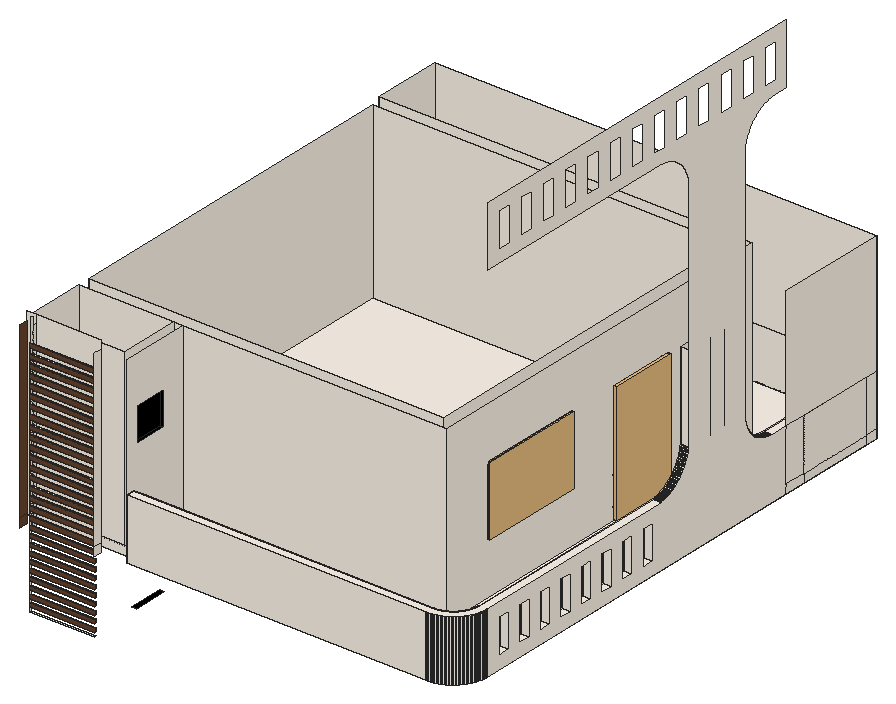
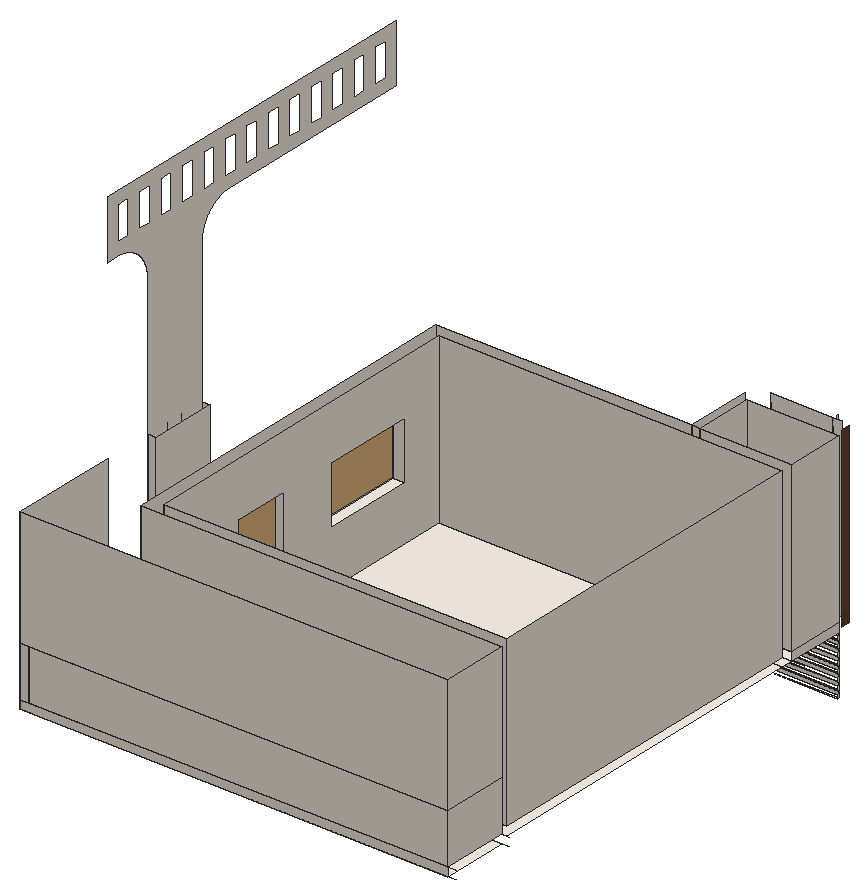
# SketchUp Ruby script. Lengths in inches.
U = 1.inch
M = Sketchup.active_model
def pt(a) = Geom::Point3d.new(a.map { |v| v * U })
def face(e, loops, mat)
  f = e.add_face(loops[0].map { |a| pt(a) })
  loops[1..].each { |l| e.add_face(l.map { |a| pt(a) }).erase! }
  f.material = f.back_material = mat if mat
  f
end
# faces: each face lists its corners as indices into pts; further lists are holes
def faces(e, pts, list, mat = nil) = list.each { |f| face(e, (f[0].is_a?(Array) ? f : [f]).map { |l| l.map { |i| pts[i] } }, mat) }
# xy, xz, yz: faces in a plane at the given z, y or x. An outline is a flat list of corners, or four numbers for a rectangle; further outlines are holes
def ring(l) = l.size == 4 ? [[l[0], l[1]], [l[2], l[1]], [l[2], l[3]], [l[0], l[3]]] : l.each_slice(2).to_a
def flat(e, list, mat, &to3) = list.each { |f| face(e, (f[0].is_a?(Array) ? f : [f]).map { |l| ring(l).map { |u, v| to3.(u, v) } }, mat) }
def xy(e, z, list, mat = nil) = flat(e, list, mat) { |x, y| [x, y, z] }
def xz(e, y, list, mat = nil) = flat(e, list, mat) { |x, z| [x, y, z] }
def yz(e, x, list, mat = nil) = flat(e, list, mat) { |y, z| [x, y, z] }
def lines(e, pts, list) = list.each { |a, b| e.add_line(pt(pts[a]), pt(pts[b])) }
# prism: a flat outline (further loops are holes) pulled along v
def prism(e, loops, v, mat = nil)
  f = face(e, loops, mat); d = Geom::Vector3d.new(v.map { |x| x * U })
  f.pushpull(f.normal.samedirection?(d) ? d.length : -d.length)
end
def box(e, o, s, mat = nil) = prism(e, [[o, [o[0] + s[0], o[1], o[2]], [o[0] + s[0], o[1] + s[1], o[2]], [o[0], o[1] + s[1], o[2]]]], [0, 0, s[2]], mat)
def at(x, y, z, deg = 0) = Geom::Transformation.translation(pt([x, y, z])) * Geom::Transformation.rotation(ORIGIN, Z_AXIS, deg.degrees)
def axes(o, x, y, z) = Geom::Transformation.new([*x, 0, *y, 0, *z, 0, *pt(o).to_a, 1])
def part(name) = M.definitions.add(name)
# library, detail: a bought-in or finely detailed component or shape, given as its bounding box
def library(name, o, s) = part(name).tap { |d| box(d.entities, o, s) }
def detail(e, o, s) = box(e.add_group.entities, o, s)
def put(e, d, t, mat = nil) = e.add_instance(d, t).tap { |i| i.material = mat if mat }
def group(e, t, mat = nil) = e.add_group.tap { |g| g.transformation = t; g.material = mat if mat }.entities
root = M.entities
M.materials.add("C01_Vanilla_Cream").color = [255, 246, 235]
M.materials.add("Wood_Veneer_15_1K").color = [103, 69, 45]
M.materials.add("[Color_009]1").color = [0, 0, 0]
c1 = library("porta+4",[0.2,-5.42,1.33],[46.55,4.72,83.21])
c2 = library("mesh-164",[-1582.71,-3144.16,-23.22],[2366.42,2227.34,65.81])
c3 = part("Group13")
put(c3.entities,c2,at(294.66,859.51,3.5))
xy(root,219.82,[[66,1,111,2]],"C01_Vanilla_Cream")
xy(root,222.5,[[66,1,111,2]],"C01_Vanilla_Cream")
xy(root,227.85,[[66,1,111,2]],"C01_Vanilla_Cream")
xy(root,230.52,[[66,1,111,2]],"C01_Vanilla_Cream")
xy(root,231,[[303,93,312,159],[303,201,312,243]],"C01_Vanilla_Cream")
xy(root,233.2,[[66,1,111,2]],"C01_Vanilla_Cream")
xy(root,235.875,[[66,1,111,2]],"C01_Vanilla_Cream")
xy(root,237.8,[[126,14.34,129,38.34]],"[Color_009]1")
xy(root,238.55,[[66,1,111,2]],"C01_Vanilla_Cream")
xy(root,241.22,[[66,1,111,2]],"C01_Vanilla_Cream")
xy(root,243.9,[[66,1,111,2]],"C01_Vanilla_Cream")
xy(root,246.58,[[66,1,111,2]],"C01_Vanilla_Cream")
xy(root,249.25,[[66,1,111,2]],"C01_Vanilla_Cream")
xy(root,251.92,[[66,1,111,2]],"C01_Vanilla_Cream")
xy(root,254.6,[[66,1,111,2]],"C01_Vanilla_Cream")
xy(root,257.27,[[66,1,111,2]],"C01_Vanilla_Cream")
xy(root,259.95,[[66,1,111,2]],"C01_Vanilla_Cream")
xy(root,262.625,[[66,1,111,2]],"C01_Vanilla_Cream")
xy(root,265.3,[[66,1,111,2]],"C01_Vanilla_Cream")
xy(root,267.98,[[66,1,111,2]],"C01_Vanilla_Cream")
xy(root,270,[[57,12,123,54],[123,12,129,54],[57,54,303,63],[303,54,312,318],[57,63,303,309],
  [54,318,303,366],[303,318,312,366]],"C01_Vanilla_Cream")
xy(root,270,[[129,6,129,54,312,54,312,366,360,366,360,30,359.99,29.25,359.95,28.49,359.89,27.74,359.8125,26.99,359.7,26.25,359.57,25.5,359.42,24.76,359.25,24.03,359.05,23.3,358.83,22.58,358.58,21.87,358.31,21.17,358.03,20.47,357.72,19.78,357.38,19.1,357.03,18.4375,356.66,17.78,356.26,17.14,355.85,16.51,355.42,15.89,354.96,15.29,354.49,14.7,354,14.13,353.5,13.57,352.97,13.03,352.43,12.5,351.87,12,351.3,11.51,350.71,11.04,350.11,10.58,349.49,10.15,348.86,9.74,348.22,9.34,347.5625,8.97,346.9,8.62,346.22,8.28,345.53,7.97,344.83,7.69,344.13,7.42,343.42,7.17,342.7,6.95,341.97,6.75,341.24,6.58,340.5,6.43,339.75,6.3,339.01,6.1875,338.26,6.11,337.51,6.05,336.75,6.01,336,6]],"Wood_Veneer_15_1K")
xy(root,270.65,[[66,1,111,2]],"C01_Vanilla_Cream")
xy(root,273.32,[[66,1,111,2]],"C01_Vanilla_Cream")
xy(root,276,[[66,1,111,2],[129,12,336,12,336.57,12.01,337.13,12.04,337.69,12.08,338.26,12.14,338.82,12.22,339.37,12.32,339.93,12.43,340.48,12.57,341.02,12.71,341.5625,12.88,342.1,13.0625,342.625,13.26,343.15,13.48,343.66,13.71,344.17,13.96,344.67,14.23,345.16,14.51,345.64,14.8,346.12,15.11,346.58,15.4375,347.03,15.78,347.47,16.13,347.9,16.5,348.32,16.88,348.73,17.27,349.12,17.68,349.5,18.1,349.87,18.53,350.22,18.97,350.5625,19.42,350.89,19.88,351.2,20.36,351.49,20.84,351.77,21.33,352.04,21.83,352.29,22.34,352.52,22.85,352.74,23.375,352.9375,23.9,353.12,24.4375,353.29,24.98,353.43,25.52,353.57,26.07,353.68,26.63,353.78,27.18,353.86,27.74,353.92,28.31,353.96,28.87,353.99,29.43,354,30,354,366,54,366,54,318,312,318,312,54,129,54],[57,12,123,54],[123,12,129,54],[57,63,303,309]],"C01_Vanilla_Cream")
xy(root,279,[[354,39,360,47.89],[354,56.78,360,65.67],[354,74.56,360,83.44],[354,92.33,360,101.22],[354,110.11,360,119],
  [354,127.89,360,136.78],[354,145.67,360,154.56],[354,163.44,360,172.33],[303,201,312,243]],"C01_Vanilla_Cream")
xy(root,279.15,[[66,1,111,2]],"C01_Vanilla_Cream")
xy(root,282.3,[[66,1,111,2]],"C01_Vanilla_Cream")
xy(root,285.45,[[66,1,111,2]],"C01_Vanilla_Cream")
xy(root,288.6,[[66,1,111,2]],"C01_Vanilla_Cream")
xy(root,291.75,[[66,1,111,2]],"C01_Vanilla_Cream")
xy(root,294.9,[[66,1,111,2]],"C01_Vanilla_Cream")
xy(root,298.05,[[66,1,111,2]],"C01_Vanilla_Cream")
xy(root,301.2,[[66,1,111,2]],"C01_Vanilla_Cream")
xy(root,303,[[354,39,360,47.89],[354,56.78,360,65.67],[354,74.56,360,83.44],[354,92.33,360,101.22],[354,110.11,360,119],
  [354,127.89,360,136.78],[354,145.67,360,154.56],[354,163.44,360,172.33]],"C01_Vanilla_Cream")
xy(root,304.35,[[66,1,111,2]],"C01_Vanilla_Cream")
xy(root,307.5,[[66,1,111,2]],"C01_Vanilla_Cream")
xy(root,310.65,[[66,1,111,2]],"C01_Vanilla_Cream")
xy(root,312,[[129,6,336,6,336.75,6.01,337.51,6.05,338.26,6.11,339.01,6.1875,339.75,6.3,340.5,6.43,341.24,6.58,341.97,6.75,342.7,6.95,343.42,7.17,344.13,7.42,344.83,7.69,345.53,7.97,346.22,8.28,346.9,8.62,347.5625,8.97,348.22,9.34,348.86,9.74,349.49,10.15,350.11,10.58,350.71,11.04,351.3,11.51,351.87,12,352.43,12.5,352.97,13.03,353.5,13.57,354,14.13,354.49,14.7,354.96,15.29,355.42,15.89,355.85,16.51,356.26,17.14,356.66,17.78,357.03,18.4375,357.38,19.1,357.72,19.78,358.03,20.47,358.31,21.17,358.58,21.87,358.83,22.58,359.05,23.3,359.25,24.03,359.42,24.76,359.57,25.5,359.7,26.25,359.8125,26.99,359.89,27.74,359.95,28.49,359.99,29.25,360,30,360,180,354,180,354,30,353.99,29.43,353.96,28.87,353.92,28.31,353.86,27.74,353.78,27.18,353.68,26.63,353.57,26.07,353.43,25.52,353.29,24.98,353.12,24.4375,352.9375,23.9,352.74,23.375,352.52,22.85,352.29,22.34,352.04,21.83,351.77,21.33,351.49,20.84,351.2,20.36,350.89,19.88,350.5625,19.42,350.22,18.97,349.87,18.53,349.5,18.1,349.12,17.68,348.73,17.27,348.32,16.88,347.9,16.5,347.47,16.13,347.03,15.78,346.58,15.4375,346.12,15.11,345.64,14.8,345.16,14.51,344.67,14.23,344.17,13.96,343.66,13.71,343.15,13.48,342.625,13.26,342.1,13.0625,341.5625,12.88,341.02,12.71,340.48,12.57,339.93,12.43,339.37,12.32,338.82,12.22,338.26,12.14,337.69,12.08,337.13,12.04,336.57,12.01,336,12,129,12],[354,276,360,366]],"C01_Vanilla_Cream")
xy(root,313.8,[[66,1,111,2]],"C01_Vanilla_Cream")
xy(root,315,[[303,93,312,159]],"C01_Vanilla_Cream")
xy(root,316.95,[[66,1,111,2]],"C01_Vanilla_Cream")
xy(root,320.1,[[66,1,111,2]],"C01_Vanilla_Cream")
xy(root,323.25,[[66,1,111,2]],"C01_Vanilla_Cream")
xy(root,326.4,[[66,1,111,2]],"C01_Vanilla_Cream")
xy(root,329.55,[[66,1,111,2]],"C01_Vanilla_Cream")
xy(root,332.7,[[66,1,111,2]],"C01_Vanilla_Cream")
xy(root,335.85,[[66,1,111,2]],"C01_Vanilla_Cream")
xy(root,339,[[66,1,111,2]],"C01_Vanilla_Cream")
xy(root,339.8,[[126,14.34,129,38.34]],"[Color_009]1")
xy(root,342.15,[[66,1,111,2]],"C01_Vanilla_Cream")
xy(root,345.3,[[66,1,111,2]],"C01_Vanilla_Cream")
xy(root,348.45,[[66,1,111,2]],"C01_Vanilla_Cream")
xy(root,351.6,[[66,1,111,2]],"C01_Vanilla_Cream")
xy(root,354.75,[[66,1,111,2]],"C01_Vanilla_Cream")
xy(root,357,[[303,93,312,159],[303,201,312,243]],"C01_Vanilla_Cream")
xy(root,357.9,[[66,1,111,2]],"C01_Vanilla_Cream")
xy(root,361.05,[[66,1,111,2]],"C01_Vanilla_Cream")
xy(root,363.8,[[126,14.34,129,38.34]],"[Color_009]1")
xy(root,364.2,[[66,1,111,2]],"C01_Vanilla_Cream")
xy(root,367.35,[[66,1,111,2]],"C01_Vanilla_Cream")
xy(root,370.5,[[66,1,111,2]],"C01_Vanilla_Cream")
xy(root,373.65,[[66,1,111,2]],"C01_Vanilla_Cream")
xy(root,376.8,[[66,1,111,2]],"C01_Vanilla_Cream")
xy(root,379.95,[[66,1,111,2]],"C01_Vanilla_Cream")
xy(root,383.1,[[66,1,111,2]],"C01_Vanilla_Cream")
xz(root,1,[[66,222.5,111,222.5,111,225.17,66,225.18],[66,227.85,111,230.52],[66,233.2,111,235.875],[66,238.55,111,241.22],[66,243.9,111,246.58],
  [66,249.25,111,251.92],[66,254.6,111,257.27],[66,259.95,111,262.625],[66,265.3,111,267.98],[66,270.65,111,273.32],
  [66,276,111,279.15],[66,282.3,111,285.45],[66,288.6,111,291.75],[66,294.9,111,298.05],[66,301.2,111,304.35],
  [66,307.5,111,310.65],[66,313.8,111,316.95],[66,320.1,111,323.25],[66,326.4,111,329.55],[66,332.7,111,335.85],
  [66,339,111,342.15],[66,345.3,111,348.45],[66,351.6,111,354.75],[66,357.9,111,361.05],[66,364.2,111,367.35],
  [66,370.5,111,373.65],[66,376.8,111,379.95],[66,383.1,111,386.25]],"Wood_Veneer_15_1K")
xz(root,2,[[66,222.5,66,225.18,111,225.17,111,222.5],[66,227.85,111,230.52],[66,233.2,111,235.875],[66,238.55,111,241.22],[66,243.9,111,246.58],
  [66,249.25,111,251.92],[66,254.6,111,257.27],[66,259.95,111,262.625],[66,265.3,111,267.98],[66,270.65,111,273.32],
  [66,276,111,279.15],[66,282.3,111,285.45],[66,288.6,111,291.75],[66,294.9,111,298.05],[66,301.2,111,304.35],
  [66,307.5,111,310.65],[66,313.8,111,316.95],[66,320.1,111,323.25],[66,326.4,111,329.55],[66,332.7,111,335.85],
  [66,339,111,342.15],[66,345.3,111,348.45],[66,351.6,111,354.75],[66,357.9,111,361.05],[66,364.2,111,367.35],
  [66,370.5,111,373.65],[66,376.8,111,379.95],[66,383.1,111,386.25]],"C01_Vanilla_Cream")
xz(root,6,[[129,270,336,312],[60,276,66,402],[66,276,111,402]],"C01_Vanilla_Cream")
xz(root,12,[[57,270,129,276],[57,276,123,396],[129,276,135,312],[135,276,336,312]],"C01_Vanilla_Cream")
xz(root,14.34,[[126,339.8,129,363.8]],"[Color_009]1")
xz(root,38.34,[[126,339.8,129,363.8]],"[Color_009]1")
xz(root,39,[[354,279,360,303]],"C01_Vanilla_Cream")
xz(root,47.89,[[354,279,360,303]],"C01_Vanilla_Cream")
xz(root,54,[[57,276,123,396],[123,276,129,396],[129,276,312,396]],"C01_Vanilla_Cream")
xz(root,56.78,[[354,279,360,303]],"C01_Vanilla_Cream")
xz(root,63,[[57,276,303,396]],"C01_Vanilla_Cream")
xz(root,65.67,[[354,279,360,303]],"C01_Vanilla_Cream")
xz(root,74.56,[[354,279,360,303]],"C01_Vanilla_Cream")
xz(root,83.44,[[354,279,360,303]],"C01_Vanilla_Cream")
xz(root,92.33,[[354,279,360,303]],"C01_Vanilla_Cream")
xz(root,93,[[303,315,312,357]],"C01_Vanilla_Cream")
xz(root,101.22,[[354,279,360,303]],"C01_Vanilla_Cream")
xz(root,110.11,[[354,279,360,303]],"C01_Vanilla_Cream")
xz(root,119,[[354,279,360,303]],"C01_Vanilla_Cream")
xz(root,127.89,[[354,279,360,303]],"C01_Vanilla_Cream")
xz(root,136.78,[[354,279,360,303]],"C01_Vanilla_Cream")
xz(root,145.67,[[354,279,360,303]],"C01_Vanilla_Cream")
xz(root,154.56,[[354,279,360,303]],"C01_Vanilla_Cream")
xz(root,159,[[303,315,312,357]],"C01_Vanilla_Cream")
xz(root,163.44,[[354,279,360,303]],"C01_Vanilla_Cream")
xz(root,172.33,[[354,279,360,303]],"C01_Vanilla_Cream")
xz(root,201,[[303,279,312,357]],"C01_Vanilla_Cream")
xz(root,204,[[354,336,360,396]],"C01_Vanilla_Cream")
xz(root,243,[[303,279,312,357]],"C01_Vanilla_Cream")
xz(root,252,[[354,336,360,396]],"C01_Vanilla_Cream")
xz(root,309,[[57,276,303,396]],"C01_Vanilla_Cream")
xz(root,318,[[54,276,312,396]],"C01_Vanilla_Cream")
xz(root,366,[[54,270,360,276],[54,276,354,312],[354,276,360,312],[54,312,360,396]],"C01_Vanilla_Cream")
yz(root,54,[[318,276,366,312],[318,312,366,396]],"C01_Vanilla_Cream")
yz(root,57,[[12,270,54,276],[12,276,54,396],[63,276,309,396]],"C01_Vanilla_Cream")
yz(root,60,[[0,270,6,276],[0,276,6,396]],"Wood_Veneer_15_1K")
yz(root,66,[[1,219.82,2,222.5],[1,225.18,2,227.85],[1,230.52,2,233.2],[1,235.875,2,238.55],[1,241.22,2,243.9],
  [1,246.58,2,249.25],[1,251.92,2,254.6],[1,257.27,2,259.95],[1,262.625,2,265.3],[1,267.98,2,270.65],
  [3,270,6,276],[1,273.32,2,276],[2,276,3,402],[3,276,6,396],[1,279.15,2,282.3],
  [1,285.45,2,288.6],[1,291.75,2,294.9],[1,298.05,2,301.2],[1,304.35,2,307.5],[1,310.65,2,313.8],
  [1,316.95,2,320.1],[1,323.25,2,326.4],[1,329.55,2,332.7],[1,335.85,2,339],[1,342.15,2,345.3],
  [1,348.45,2,351.6],[1,354.75,2,357.9],[1,361.05,2,364.2],[1,367.35,2,370.5],[1,373.65,2,376.8],
  [1,379.95,2,383.1]],"C01_Vanilla_Cream")
yz(root,111,[[[0,270,6,276],[1,270.65,2,273.32]],[[0,276,0,396,1,396,1,395.7,2,395.7,2,396,6,396,6,276,2,276,2,279.15,1,279.15,1,276],[1,326.4,2,329.55],[1,301.2,2,304.35],[1,294.9,2,298.05],[1,389.4,2,392.55],[1,383.1,2,386.25],[1,376.8,2,379.95],[1,370.5,2,373.65],[1,364.2,2,367.35],[1,357.9,2,361.05],[1,351.6,2,354.75],[1,345.3,2,348.45],[1,339,2,342.15],[1,332.7,2,335.85],[1,320.1,2,323.25],[1,313.8,2,316.95],[1,307.5,2,310.65],[1,288.6,2,291.75],[1,282.3,2,285.45]]],"C01_Vanilla_Cream")
yz(root,123,[[12,276,54,396]],"C01_Vanilla_Cream")
yz(root,126,[[14.34,339.8,38.34,363.8]],"[Color_009]1")
yz(root,129,[[6,270,12,276],[6,276,12,312],[[12,276,54,276,54,396,6,396,6,312,12,312],[14.34,339.8,38.34,363.8]]],"C01_Vanilla_Cream")
yz(root,303,[[[63,276,309,396],[201,279,243,357],[93,315,159,357]]],"C01_Vanilla_Cream")
yz(root,312,[[[54,276,198,276,198,360,246,360,246,276,318,276,318,396,54,396],[90,312,162,360]],[[198,276,246,360],[201,279,243,357]],[[90,312,162,360],[93,315,159,357]]],"C01_Vanilla_Cream")
yz(root,354,[[[30,276,30,312,180,312,180.72,312.11,181.44,312.23,182.16,312.375,182.87,312.54,183.57,312.72,184.28,312.92,184.97,313.13,185.66,313.37,186.35,313.62,187.02,313.89,187.69,314.18,188.36,314.49,189.01,314.8125,189.66,315.15,190.29,315.51,190.92,315.88,191.54,316.27,192.14,316.68,192.74,317.1,193.32,317.53,193.89,317.99,194.45,318.45,195,318.93,195.54,319.43,196.0625,319.9375,196.57,320.46,197.07,321,197.55,321.55,198.01,322.11,198.47,322.68,198.9,323.26,199.32,323.86,199.73,324.46,200.12,325.08,200.49,325.71,200.85,326.34,201.1875,326.99,201.51,327.64,201.82,328.31,202.11,328.98,202.38,329.65,202.63,330.34,202.87,331.03,203.08,331.72,203.28,332.43,203.46,333.13,203.625,333.84,203.77,334.56,203.89,335.28,204,336,204,396,252,396,252,336,252.01,335.25,252.05,334.49,252.11,333.74,252.2,332.99,252.3,332.25,252.43,331.51,252.59,330.77,252.77,330.04,252.97,329.3125,253.1875,328.59,253.43,327.88,253.7,327.17,253.99,326.48,254.3,325.79,254.63,325.12,254.99,324.45,255.36,323.8,255.75,323.15,256.17,322.52,256.6,321.91,257.06,321.31,257.53,320.72,258.02,320.15,258.52,319.59,259.05,319.05,259.59,318.52,260.15,318.02,260.72,317.53,261.31,317.06,261.91,316.6,262.52,316.17,263.15,315.75,263.8,315.36,264.45,314.99,265.12,314.63,265.79,314.3,266.48,313.99,267.17,313.7,267.88,313.43,268.59,313.1875,269.3125,312.97,270.04,312.77,270.77,312.59,271.51,312.43,272.25,312.3,272.99,312.2,273.74,312.11,274.49,312.05,275.25,312.01,276,312,366,312,366,276],[39,279,47.89,303],[56.78,279,65.67,303],[92.33,279,101.22,303],[110.11,279,119,303],[127.89,279,136.78,303],[163.44,279,172.33,303],[74.56,279,83.44,303],[145.67,279,154.56,303]]],"C01_Vanilla_Cream")
yz(root,360,[[[30,270,288,270,288,312,276,312,275.25,312.01,274.49,312.05,273.74,312.11,272.99,312.2,272.25,312.3,271.51,312.43,270.77,312.59,270.04,312.77,269.3125,312.97,268.59,313.1875,267.88,313.43,267.17,313.7,266.48,313.99,265.79,314.3,265.12,314.63,264.45,314.99,263.8,315.36,263.15,315.75,262.52,316.17,261.91,316.6,261.31,317.06,260.72,317.53,260.15,318.02,259.59,318.52,259.05,319.05,258.52,319.59,258.02,320.15,257.53,320.72,257.06,321.31,256.6,321.91,256.17,322.52,255.75,323.15,255.36,323.8,254.99,324.45,254.63,325.12,254.3,325.79,253.99,326.48,253.7,327.17,253.43,327.88,253.1875,328.59,252.97,329.3125,252.77,330.04,252.59,330.77,252.43,331.51,252.3,332.25,252.2,332.99,252.11,333.74,252.05,334.49,252.01,335.25,252,336,252,498,252.08,498.73,252.18,499.46,252.29,500.1875,252.43,500.91,252.59,501.63,252.77,502.35,252.97,503.06,253.18,503.76,253.42,504.46,253.68,505.15,253.95,505.83,254.25,506.5,254.56,507.17,254.89,507.83,255.24,508.48,255.61,509.12,255.99,509.74,256.39,510.36,256.8125,510.97,257.25,511.56,257.7,512.14,258.17,512.71,258.65,513.27,259.15,513.81,259.66,514.34,260.19,514.85,260.73,515.35,261.29,515.83,261.86,516.3,262.44,516.75,263.03,517.1875,263.64,517.61,264.26,518.01,264.88,518.39,265.52,518.76,266.17,519.11,266.83,519.44,267.5,519.75,268.17,520.05,268.85,520.32,269.54,520.58,270.24,520.82,270.94,521.03,271.65,521.23,272.37,521.41,273.09,521.57,273.8125,521.71,274.54,521.82,275.27,521.92,276,522,288,522,288,564,30,564,30,522,180,522,180.75,521.96,181.49,521.9,182.23,521.82,182.97,521.71,183.71,521.58,184.4375,521.44,185.16,521.26,185.89,521.07,186.6,520.86,187.31,520.62,188.01,520.36,188.7,520.09,189.39,519.79,190.0625,519.47,190.73,519.13,191.38,518.77,192.03,518.39,192.66,518,193.28,517.58,193.89,517.15,194.48,516.69,195.0625,516.22,195.625,515.74,196.18,515.23,196.71,514.71,197.23,514.18,197.74,513.625,198.22,513.0625,198.69,512.48,199.15,511.89,199.58,511.28,200,510.66,200.39,510.03,200.77,509.38,201.13,508.73,201.47,508.0625,201.79,507.39,202.09,506.7,202.36,506.01,202.62,505.31,202.86,504.6,203.07,503.89,203.26,503.16,203.44,502.4375,203.58,501.71,203.71,500.97,203.82,500.23,203.9,499.49,203.96,498.75,204,498,204,336,203.89,335.28,203.77,334.56,203.625,333.84,203.46,333.13,203.28,332.43,203.08,331.72,202.87,331.03,202.63,330.34,202.38,329.65,202.11,328.98,201.82,328.31,201.51,327.64,201.1875,326.99,200.85,326.34,200.49,325.71,200.12,325.08,199.73,324.46,199.32,323.86,198.9,323.26,198.47,322.68,198.01,322.11,197.55,321.55,197.07,321,196.57,320.46,196.0625,319.9375,195.54,319.43,195,318.93,194.45,318.45,193.89,317.99,193.32,317.53,192.74,317.1,192.14,316.68,191.54,316.27,190.92,315.88,190.29,315.51,189.66,315.15,189.01,314.8125,188.36,314.49,187.69,314.18,187.02,313.89,186.35,313.62,185.66,313.37,184.97,313.13,184.28,312.92,183.57,312.72,182.87,312.54,182.16,312.375,181.44,312.23,180.72,312.11,180,312,30,312],[96.6,531,106.2,555],[115.8,531,125.4,555],[192.6,531,202.2,555],[269.4,531,279,555],[250.2,531,259.8,555],[39,531,48.6,555],[58.2,531,67.8,555],[77.4,531,87,555],[135,531,144.6,555],[154.2,531,163.8,555],[173.4,531,183,555],[211.8,531,221.4,555],[231,531,240.6,555],[39,279,47.89,303],[56.78,279,65.67,303],[110.11,279,119,303],[92.33,279,101.22,303],[127.89,279,136.78,303],[163.44,279,172.33,303],[74.56,279,83.44,303],[145.67,279,154.56,303]],[288,270,303,276],[303,270,357,276],[357,270,366,276],[288,276,303,312],
  [303,276,357,312],[357,276,366,312],[288,312,366,396]],"C01_Vanilla_Cream")
p = [[66,2,225.18],[66,1,225.18],[111,1,225.17],[111,2,225.17],[336.75,6.01,270],[336.75,6.01,312],
  [336,6,312],[336,6,270],[337.51,6.05,270],[337.51,6.05,312],[338.26,6.11,270],[338.26,6.11,312],
  [339.01,6.1875,270],[339.01,6.1875,312],[339.75,6.3,270],[339.75,6.3,312],[340.5,6.43,270],[340.5,6.43,312],
  [341.24,6.58,270],[341.24,6.58,312],[341.97,6.75,270],[341.97,6.75,312],[342.7,6.95,270],[342.7,6.95,312],
  [343.42,7.17,270],[343.42,7.17,312],[344.13,7.42,270],[344.13,7.42,312],[344.83,7.69,270],[344.83,7.69,312],
  [345.53,7.97,270],[345.53,7.97,312],[346.22,8.28,270],[346.22,8.28,312],[346.9,8.62,270],[346.9,8.62,312],
  [347.5625,8.97,270],[347.5625,8.97,312],[348.22,9.34,270],[348.22,9.34,312],[348.86,9.74,270],[348.86,9.74,312],
  [349.49,10.15,270],[349.49,10.15,312],[350.11,10.58,270],[350.11,10.58,312],[350.71,11.04,270],[350.71,11.04,312],
  [351.3,11.51,270],[351.3,11.51,312],[351.87,12,270],[351.87,12,312],[352.43,12.5,270],[352.43,12.5,312],
  [352.97,13.03,270],[352.97,13.03,312],[353.5,13.57,270],[353.5,13.57,312],[354,14.13,270],[354,14.13,312],
  [354.49,14.7,270],[354.49,14.7,312],[354.96,15.29,270],[354.96,15.29,312],[355.42,15.89,270],[355.42,15.89,312],
  [355.85,16.51,270],[355.85,16.51,312],[356.26,17.14,270],[356.26,17.14,312],[356.66,17.78,270],[356.66,17.78,312],
  [357.03,18.4375,270],[357.03,18.4375,312],[357.38,19.1,270],[357.38,19.1,312],[357.72,19.78,270],[357.72,19.78,312],
  [358.03,20.47,270],[358.03,20.47,312],[358.31,21.17,270],[358.31,21.17,312],[358.58,21.87,270],[358.58,21.87,312],
  [358.83,22.58,270],[358.83,22.58,312],[359.05,23.3,270],[359.05,23.3,312],[359.25,24.03,270],[359.25,24.03,312],
  [359.42,24.76,270],[359.42,24.76,312],[359.57,25.5,270],[359.57,25.5,312],[359.7,26.25,270],[359.7,26.25,312],
  [359.8125,26.99,270],[359.8125,26.99,312],[359.89,27.74,270],[359.89,27.74,312],[359.95,28.49,270],[359.95,28.49,312],
  [359.99,29.25,270],[359.99,29.25,312],[360,30,270],[360,30,312],[336.57,12.01,276],[336,12,276],
  [336,12,312],[336.57,12.01,312],[337.13,12.04,276],[337.13,12.04,312],[337.69,12.08,276],[337.69,12.08,312],
  [338.26,12.14,276],[338.26,12.14,312],[338.82,12.22,276],[338.82,12.22,312],[339.37,12.32,276],[339.37,12.32,312],
  [339.93,12.43,276],[339.93,12.43,312],[340.48,12.57,276],[340.48,12.57,312],[341.02,12.71,276],[341.02,12.71,312],
  [341.5625,12.88,276],[341.5625,12.88,312],[342.1,13.0625,276],[342.1,13.0625,312],[342.625,13.26,276],[342.625,13.26,312],
  [343.15,13.48,276],[343.15,13.48,312],[343.66,13.71,276],[343.66,13.71,312],[344.17,13.96,276],[344.17,13.96,312],
  [344.67,14.23,276],[344.67,14.23,312],[345.16,14.51,276],[345.16,14.51,312],[345.64,14.8,276],[345.64,14.8,312],
  [346.12,15.11,276],[346.12,15.11,312],[346.58,15.4375,276],[346.58,15.4375,312],[347.03,15.78,276],[347.03,15.78,312],
  [347.47,16.13,276],[347.47,16.13,312],[347.9,16.5,276],[347.9,16.5,312],[348.32,16.88,276],[348.32,16.88,312],
  [348.73,17.27,276],[348.73,17.27,312],[349.12,17.68,276],[349.12,17.68,312],[349.5,18.1,276],[349.5,18.1,312],
  [349.87,18.53,276],[349.87,18.53,312],[350.22,18.97,276],[350.22,18.97,312],[350.5625,19.42,276],[350.5625,19.42,312],
  [350.89,19.88,276],[350.89,19.88,312],[351.2,20.36,276],[351.2,20.36,312],[351.49,20.84,276],[351.49,20.84,312],
  [351.77,21.33,276],[351.77,21.33,312],[352.04,21.83,276],[352.04,21.83,312],[352.29,22.34,276],[352.29,22.34,312],
  [352.52,22.85,276],[352.52,22.85,312],[352.74,23.375,276],[352.74,23.375,312],[352.9375,23.9,276],[352.9375,23.9,312],
  [353.12,24.4375,276],[353.12,24.4375,312],[353.29,24.98,276],[353.29,24.98,312],[353.43,25.52,276],[353.43,25.52,312],
  [353.57,26.07,276],[353.57,26.07,312],[353.68,26.63,276],[353.68,26.63,312],[353.78,27.18,276],[353.78,27.18,312],
  [353.86,27.74,276],[353.86,27.74,312],[353.92,28.31,276],[353.92,28.31,312],[353.96,28.87,276],[353.96,28.87,312],
  [353.99,29.43,276],[353.99,29.43,312],[354,30,276],[354,30,312],[360,180,312],[360,180.72,312.11],
  [354,180.72,312.11],[354,180,312],[360,274.49,312.05],[360,275.25,312.01],[354,275.25,312.01],[354,274.49,312.05],
  [360,276,312],[354,276,312],[360,181.44,312.23],[354,181.44,312.23],[360,272.99,312.2],[360,273.74,312.11],
  [354,273.74,312.11],[354,272.99,312.2],[360,182.16,312.375],[354,182.16,312.375],[360,272.25,312.3],[354,272.25,312.3],
  [360,271.51,312.43],[354,271.51,312.43],[360,182.87,312.54],[354,182.87,312.54],[360,270.77,312.59],[354,270.77,312.59],
  [360,183.57,312.72],[354,183.57,312.72],[360,270.04,312.77],[354,270.04,312.77],[360,184.28,312.92],[354,184.28,312.92],
  [360,269.3125,312.97],[354,269.3125,312.97],[360,184.97,313.13],[354,184.97,313.13],[360,268.59,313.1875],[354,268.59,313.1875],
  [360,185.66,313.37],[354,185.66,313.37],[360,267.88,313.43],[354,267.88,313.43],[360,186.35,313.62],[354,186.35,313.62],
  [360,267.17,313.7],[354,267.17,313.7],[360,187.02,313.89],[354,187.02,313.89],[360,266.48,313.99],[354,266.48,313.99],
  [360,187.69,314.18],[354,187.69,314.18],[360,265.79,314.3],[354,265.79,314.3],[360,188.36,314.49],[354,188.36,314.49],
  [360,265.12,314.63],[354,265.12,314.63],[360,189.01,314.8125],[354,189.01,314.8125],[360,264.45,314.99],[354,264.45,314.99],
  [360,189.66,315.15],[354,189.66,315.15],[360,263.8,315.36],[354,263.8,315.36],[360,190.29,315.51],[354,190.29,315.51],
  [360,263.15,315.75],[354,263.15,315.75],[360,190.92,315.88],[354,190.92,315.88],[360,262.52,316.17],[354,262.52,316.17],
  [360,191.54,316.27],[354,191.54,316.27],[360,261.91,316.6],[354,261.91,316.6],[360,192.14,316.68],[354,192.14,316.68],
  [360,261.31,317.06],[354,261.31,317.06],[360,192.74,317.1],[354,192.74,317.1],[360,193.32,317.53],[354,193.32,317.53],
  [360,260.72,317.53],[354,260.72,317.53],[360,193.89,317.99],[354,193.89,317.99],[360,260.15,318.02],[354,260.15,318.02],
  [360,194.45,318.45],[354,194.45,318.45],[360,259.59,318.52],[354,259.59,318.52],[360,195,318.93],[354,195,318.93],
  [360,259.05,319.05],[354,259.05,319.05],[360,195.54,319.43],[354,195.54,319.43],[360,258.52,319.59],[354,258.52,319.59],
  [360,196.0625,319.9375],[354,196.0625,319.9375],[360,258.02,320.15],[354,258.02,320.15],[360,196.57,320.46],[354,196.57,320.46],
  [360,257.53,320.72],[354,257.53,320.72],[360,197.07,321],[354,197.07,321],[360,257.06,321.31],[354,257.06,321.31],
  [360,197.55,321.55],[354,197.55,321.55],[360,256.6,321.91],[354,256.6,321.91],[360,198.01,322.11],[354,198.01,322.11],
  [360,256.17,322.52],[354,256.17,322.52],[360,198.47,322.68],[354,198.47,322.68],[360,255.75,323.15],[354,255.75,323.15],
  [360,198.9,323.26],[354,198.9,323.26],[360,255.36,323.8],[354,255.36,323.8],[360,199.32,323.86],[354,199.32,323.86],
  [360,254.99,324.45],[354,254.99,324.45],[360,199.73,324.46],[354,199.73,324.46],[360,200.12,325.08],[354,200.12,325.08],
  [360,254.63,325.12],[354,254.63,325.12],[360,200.49,325.71],[354,200.49,325.71],[360,254.3,325.79],[354,254.3,325.79],
  [360,200.85,326.34],[354,200.85,326.34],[360,253.99,326.48],[354,253.99,326.48],[360,201.1875,326.99],[354,201.1875,326.99],
  [360,253.7,327.17],[354,253.7,327.17],[360,201.51,327.64],[354,201.51,327.64],[360,253.43,327.88],[354,253.43,327.88],
  [360,201.82,328.31],[354,201.82,328.31],[360,253.1875,328.59],[354,253.1875,328.59],[360,202.11,328.98],[354,202.11,328.98],
  [360,252.97,329.3125],[354,252.97,329.3125],[360,202.38,329.65],[354,202.38,329.65],[360,252.77,330.04],[354,252.77,330.04],
  [360,202.63,330.34],[354,202.63,330.34],[360,252.59,330.77],[354,252.59,330.77],[360,202.87,331.03],[354,202.87,331.03],
  [360,252.43,331.51],[354,252.43,331.51],[360,203.08,331.72],[354,203.08,331.72],[360,252.3,332.25],[354,252.3,332.25],
  [360,203.28,332.43],[354,203.28,332.43],[360,252.2,332.99],[354,252.2,332.99],[360,203.46,333.13],[354,203.46,333.13],
  [360,252.11,333.74],[354,252.11,333.74],[360,203.625,333.84],[354,203.625,333.84],[360,252.05,334.49],[354,252.05,334.49],
  [360,203.77,334.56],[354,203.77,334.56],[360,252.01,335.25],[354,252.01,335.25],[360,203.89,335.28],[354,203.89,335.28],
  [360,252,336],[354,252,336],[360,204,336],[354,204,336],[48,54,270],[57,54,270],
  [48,318,276],[54,318,276],[135,48,276],[135,12,276],[360,222,396],[360,222,335.34],
  [360,234,335.98],[360,234,396],[54,366,276],[48,366,276],[54,366,270],[48,366,270],
  [54,318,270],[48,318,270]]
faces(root,p,[[0,1,2,3],[4,5,6,7],[8,9,5,4],[10,11,9,8],[12,13,11,10],[14,15,13,12],[16,17,15,14],[18,19,17,16],
  [20,21,19,18],[22,23,21,20],[24,25,23,22],[26,27,25,24],[28,29,27,26],[30,31,29,28],[32,33,31,30],[34,35,33,32],
  [36,37,35,34],[38,39,37,36],[40,41,39,38],[42,43,41,40],[44,45,43,42],[46,47,45,44],[48,49,47,46],[50,51,49,48],
  [52,53,51,50],[54,55,53,52],[56,57,55,54],[58,59,57,56],[60,61,59,58],[62,63,61,60],[64,65,63,62],[66,67,65,64],
  [68,69,67,66],[70,71,69,68],[72,73,71,70],[74,75,73,72],[76,77,75,74],[78,79,77,76],[80,81,79,78],[82,83,81,80],
  [84,85,83,82],[86,87,85,84],[88,89,87,86],[90,91,89,88],[92,93,91,90],[94,95,93,92],[96,97,95,94],[98,99,97,96],
  [100,101,99,98],[102,103,101,100],[104,105,103,102],[106,107,108,109],[110,106,109,111],[112,110,111,113],[114,112,113,115],[116,114,115,117],
  [118,116,117,119],[120,118,119,121],[122,120,121,123],[124,122,123,125],[126,124,125,127],[128,126,127,129],[130,128,129,131],[132,130,131,133],
  [134,132,133,135],[136,134,135,137],[138,136,137,139],[140,138,139,141],[142,140,141,143],[144,142,143,145],[146,144,145,147],[148,146,147,149],
  [150,148,149,151],[152,150,151,153],[154,152,153,155],[156,154,155,157],[158,156,157,159],[160,158,159,161],[162,160,161,163],[164,162,163,165],
  [166,164,165,167],[168,166,167,169],[170,168,169,171],[172,170,171,173],[174,172,173,175],[176,174,175,177],[178,176,177,179],[180,178,179,181],
  [182,180,181,183],[184,182,183,185],[186,184,185,187],[188,186,187,189],[190,188,189,191],[192,190,191,193],[194,192,193,195],[196,194,195,197],
  [198,196,197,199],[200,198,199,201],[202,200,201,203],[204,202,203,205],[206,204,205,207],[208,209,210,211],[212,213,214,215],[213,216,217,214],
  [209,218,219,210],[220,221,222,223],[221,212,215,222],[218,224,225,219],[226,220,223,227],[228,226,227,229],[224,230,231,225],[232,228,229,233],
  [230,234,235,231],[236,232,233,237],[234,238,239,235],[240,236,237,241],[238,242,243,239],[244,240,241,245],[242,246,247,243],[248,244,245,249],
  [246,250,251,247],[252,248,249,253],[250,254,255,251],[256,252,253,257],[254,258,259,255],[260,256,257,261],[258,262,263,259],[264,260,261,265],
  [262,266,267,263],[268,264,265,269],[266,270,271,267],[272,268,269,273],[270,274,275,271],[276,272,273,277],[274,278,279,275],[280,276,277,281],
  [278,282,283,279],[284,280,281,285],[282,286,287,283],[288,284,285,289],[286,290,291,287],[290,292,293,291],[294,288,289,295],[292,296,297,293],
  [298,294,295,299],[296,300,301,297],[302,298,299,303],[300,304,305,301],[306,302,303,307],[304,308,309,305],[310,306,307,311],[308,312,313,309],
  [314,310,311,315],[312,316,317,313],[318,314,315,319],[316,320,321,317],[322,318,319,323],[320,324,325,321],[326,322,323,327],[324,328,329,325],
  [330,326,327,331],[328,332,333,329],[334,330,331,335],[332,336,337,333],[338,334,335,339],[336,340,341,337],[342,338,339,343],[340,344,345,341],
  [344,346,347,345],[348,342,343,349],[346,350,351,347],[352,348,349,353],[350,354,355,351],[356,352,353,357],[354,358,359,355],[360,356,357,361],
  [358,362,363,359],[364,360,361,365],[362,366,367,363],[368,364,365,369],[366,370,371,367],[372,368,369,373],[370,374,375,371],[376,372,373,377],
  [374,378,379,375],[380,376,377,381],[378,382,383,379],[384,380,381,385],[382,386,387,383],[388,384,385,389],[386,390,391,387],[392,388,389,393],
  [390,394,395,391],[396,392,393,397],[394,398,399,395],[400,396,397,401],[398,402,403,399],[404,400,401,405],[402,406,407,403],[408,404,405,409],
  [406,410,411,407]],"C01_Vanilla_Cream")
lines(root,p,[[412,413],[414,415],[416,417],[418,419],[420,421],[422,423],[424,425],[426,427]])
put(root,c1,at(309.24,197.8,275.48,90))
put(root,c3,axes([312.39,129.3,361.23],[0,0.03051,0],[0,0,0.02146],[0.01969,0,0]))
